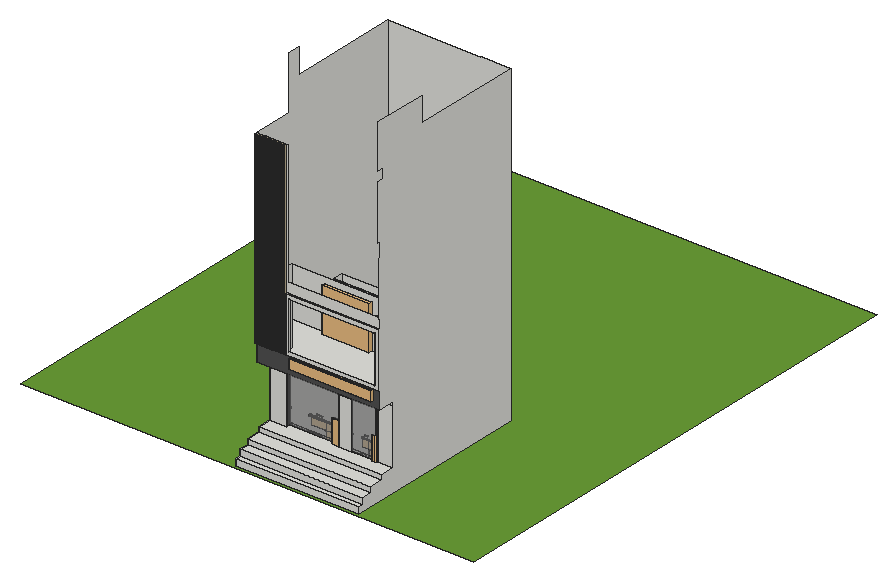
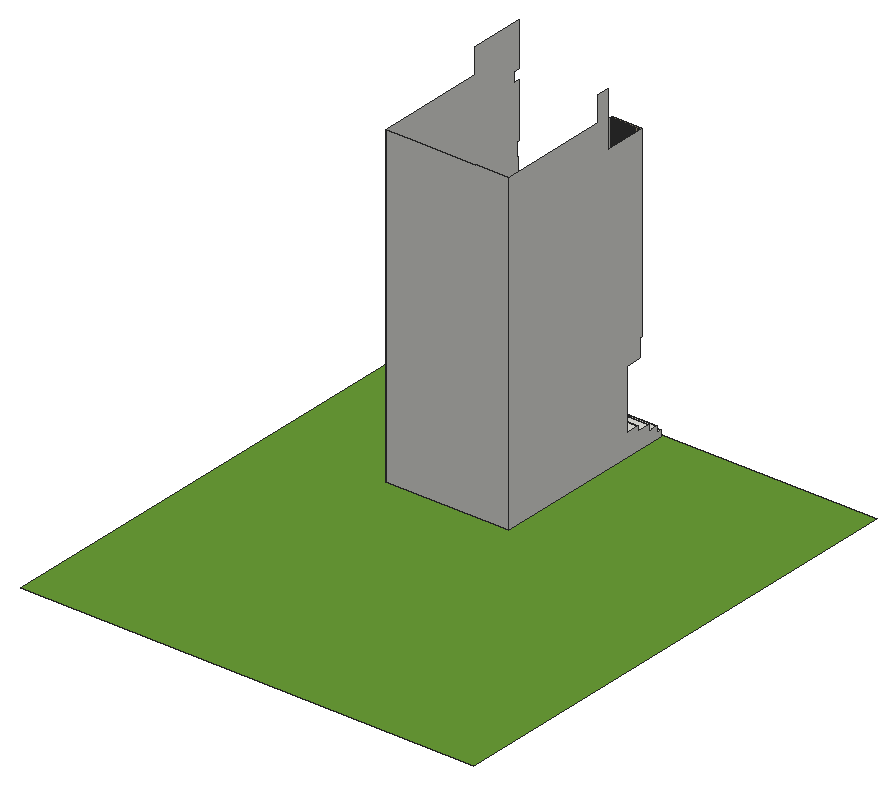
# SketchUp Ruby script. Lengths in inches.
U = 1.inch
M = Sketchup.active_model
def pt(a) = Geom::Point3d.new(a.map { |v| v * U })
def face(e, loops, mat)
  f = e.add_face(loops[0].map { |a| pt(a) })
  loops[1..].each { |l| e.add_face(l.map { |a| pt(a) }).erase! }
  f.material = f.back_material = mat if mat
  f
end
# faces: each face lists its corners as indices into pts; further lists are holes
def faces(e, pts, list, mat = nil) = list.each { |f| face(e, (f[0].is_a?(Array) ? f : [f]).map { |l| l.map { |i| pts[i] } }, mat) }
# xy, xz, yz: faces in a plane at the given z, y or x. An outline is a flat list of corners, or four numbers for a rectangle; further outlines are holes
def ring(l) = l.size == 4 ? [[l[0], l[1]], [l[2], l[1]], [l[2], l[3]], [l[0], l[3]]] : l.each_slice(2).to_a
def flat(e, list, mat, &to3) = list.each { |f| face(e, (f[0].is_a?(Array) ? f : [f]).map { |l| ring(l).map { |u, v| to3.(u, v) } }, mat) }
def xy(e, z, list, mat = nil) = flat(e, list, mat) { |x, y| [x, y, z] }
def xz(e, y, list, mat = nil) = flat(e, list, mat) { |x, z| [x, y, z] }
def yz(e, x, list, mat = nil) = flat(e, list, mat) { |y, z| [x, y, z] }
def lines(e, pts, list) = list.each { |a, b| e.add_line(pt(pts[a]), pt(pts[b])) }
# prism: a flat outline (further loops are holes) pulled along v
def prism(e, loops, v, mat = nil)
  f = face(e, loops, mat); d = Geom::Vector3d.new(v.map { |x| x * U })
  f.pushpull(f.normal.samedirection?(d) ? d.length : -d.length)
end
def box(e, o, s, mat = nil) = prism(e, [[o, [o[0] + s[0], o[1], o[2]], [o[0] + s[0], o[1] + s[1], o[2]], [o[0], o[1] + s[1], o[2]]]], [0, 0, s[2]], mat)
def at(x, y, z, deg = 0) = Geom::Transformation.translation(pt([x, y, z])) * Geom::Transformation.rotation(ORIGIN, Z_AXIS, deg.degrees)
def axes(o, x, y, z) = Geom::Transformation.new([*x, 0, *y, 0, *z, 0, *pt(o).to_a, 1])
def part(name) = M.definitions.add(name)
# library, detail: a bought-in or finely detailed component or shape, given as its bounding box
def library(name, o, s) = part(name).tap { |d| box(d.entities, o, s) }
def detail(e, o, s) = box(e.add_group.entities, o, s)
def put(e, d, t, mat = nil) = e.add_instance(d, t).tap { |i| i.material = mat if mat }
def group(e, t, mat = nil) = e.add_group.tap { |g| g.transformation = t; g.material = mat if mat }.entities
root = M.entities
M.materials.add("SW 0012 Empire Gold").color = [192, 162, 108]
M.materials.add("SW 0028 Caen Stone").color = [234, 212, 175]
M.materials.add("SW 0030 Colonial Yellow").color = [235, 202, 133]
M.materials.add("SW 0044 Hubbard Squash").color = [228, 196, 137]
M.materials.add("SW 0067 Belvedere Cream").color = [236, 208, 158]
M.materials.add("SW 0078 Sunbeam Yellow").color = [236, 216, 155]
M.materials.add("SW 2834 Birdseye Maple").color = [221, 199, 142]
M.materials.add("SW 2853 New Colonial Yellow").color = [211, 178, 125]
M.materials.add("SW 2857 Peace Yellow").color = [231, 210, 153]
M.materials.add("SW 2865 Classical Yellow").color = [244, 218, 144]
M.materials.add("SW 6113 Interactive Cream").color = [226, 206, 173]
M.materials.add("SW 6114 Bagel").color = [213, 185, 146]
M.materials.add("SW 6115 Totally Tan").color = [202, 170, 129]
M.materials.add("SW 6120 Believable Buff").color = [216, 202, 167]
M.materials.add("SW 6121 Whole Wheat").color = [203, 185, 145]
M.materials.add("SW 6122 Camelback").color = [194, 175, 133]
M.materials.add("SW 6127 Ivoire").color = [224, 209, 170]
M.materials.add("SW 6128 Blonde").color = [217, 193, 145]
M.materials.add("SW 6129 Restrained Gold").color = [206, 183, 131]
M.materials.add("SW 6134 Netsuke").color = [220, 210, 175]
M.materials.add("SW 6135 Ecru").color = [206, 193, 149]
M.materials.add("SW 6136 Harmonic Tan").color = [194, 179, 136]
M.materials.add("SW 6365 Cachet Cream").color = [240, 220, 183]
M.materials.add("SW 6366 Ambitious Amber").color = [238, 208, 148]
M.materials.add("SW 6372 Inviting Ivory").color = [239, 218, 175]
M.materials.add("SW 6373 Harvester").color = [232, 201, 137]
M.materials.add("SW 6379 Jersey Cream").color = [239, 224, 185]
M.materials.add("SW 6380 Humble Gold").color = [232, 206, 147]
M.materials.add("SW 6387 Compatible Cream").color = [229, 206, 156]
M.materials.add("SW 6388 Golden Fleece").color = [227, 182, 114]
M.materials.add("SW 6393 Convivial Yellow").color = [229, 218, 173]
M.materials.add("SW 6394 Sequin").color = [220, 200, 139]
M.materials.add("SW 6400 Lucent Yellow").color = [223, 213, 164]
M.materials.add("SW 6407 Ancestral Gold").color = [218, 210, 164]
M.materials.add("SW 6659 Captivating Cream").color = [243, 220, 176]
M.materials.add("SW 6660 Honey Blush").color = [243, 211, 152]
M.materials.add("SW 6666 Enjoyable Yellow").color = [244, 218, 167]
M.materials.add("SW 6667 Afterglow").color = [243, 209, 138]
M.materials.add("SW 6673 Banana Cream").color = [243, 226, 174]
M.materials.add("SW 6674 Jonquil").color = [244, 216, 142]
M.materials.add("SW 6680 Friendly Yellow").color = [241, 228, 176]
M.materials.add("SW 6681 Butter Up").color = [243, 225, 159]
M.materials.add("SW 6687 Lantern Light").color = [241, 228, 173]
M.materials.add("SW 6688 Solaria").color = [242, 221, 140]
M.materials.add("SW 6694 Glad Yellow").color = [240, 230, 169]
M.materials.add("SW 6701 Moonraker").color = [234, 231, 176]
M.materials.add("SW 6888 Pizazz Peach").color = [243, 202, 146]
M.materials.add("SW 6896 Solé").color = [243, 226, 157]
M.materials.add("SW 6900 Optimistic Yellow").color = [242, 228, 163]
M.materials.add("SW 6908 Fun Yellow").color = [242, 235, 145]
M.materials.add("SW 6912 Glisten Yellow").color = [240, 235, 169]
M.materials.add("SW 7537 Irish Cream").color = [227, 211, 186]
M.materials.add("SW 7676 Paper Lantern").color = [240, 224, 198]
M.materials.add("SW 7677 Gold Vessel").color = [233, 187, 138]
M.materials.add("SW 7678 Cottage Cream").color = [236, 219, 189]
M.materials.add("SW 7679 Golden Gate").color = [217, 176, 132]
M.materials.add("SW 7680 Lanyard").color = [191, 153, 116]
M.materials.add("SW 7681 Tea Light").color = [246, 227, 194]
M.materials.add("SW 7682 Bee_s Wax").color = [233, 192, 136]
M.materials.add("SW 7683 Buff").color = [242, 225, 197]
M.materials.add("SW 7684 Concord Buff").color = [239, 216, 182]
M.materials.add("SW 7685 White Raisin").color = [228, 192, 140]
M.materials.add("SW 7686 Hinoki").color = [246, 220, 183]
M.materials.add("SW 7687 August Moon").color = [231, 199, 161]
M.materials.add("SW 7688 Sundew").color = [223, 206, 176]
M.materials.add("SW 7689 Row House Tan").color = [211, 187, 159]
M.materials.add("SW 7690 Townhall Tan").color = [194, 171, 140]
M.materials.add("SW 7691 Biltmore Buff").color = [225, 202, 161]
M.materials.add("SW 7692 Cupola Yellow").color = [219, 188, 144]
M.materials.add("SW 7693 Stonebriar").color = [203, 172, 128]
M.materials.add("SW 7694 Dromedary Camel").color = [203, 175, 136]
M.materials.add("SW 7695 Mesa Tan").color = [190, 160, 124]
M.materials.add("SW 7696 Toasted Pine Nut").color = [218, 199, 167]
M.materials.add("SW 7697 Safari").color = [203, 179, 141]
M.materials.add("SW 7698 Straw Harvest").color = [217, 199, 161]
M.materials.add("SW 7717 Ligonier Tan").color = [211, 178, 143]
M.materials.add("Translucent_Glass_Gray1").color = [128, 128, 128]
M.materials["Translucent_Glass_Gray1"].alpha = 0.37
M.materials.add("[0010_Snow]").color = [255, 250, 250]
M.materials.add("[0135_DarkGray]").color = [81, 81, 81]
M.materials.add("[Color I05]").color = [0, 0, 255]
M.materials.add("[Grass Dark Green]").color = [106, 157, 55]
M.materials.add("[Quartz Light Brown]").color = [199, 184, 152]
M.materials.add("[Wax 01]").color = [250, 213, 163]
c1 = library("AED Menu Board with Easel",[149.1875,-32.32,34.05],[43.29,34.63,95.15])
c2 = part("Metal Door Roller Shutter")
xy(c2.entities,0,[[0,-0.5,0,4.5625,58.5,4.5625,58.5,-0.5,56.37,-0.5,56.37,1.125,1.83,1.125,1.83,-0.5]])
xy(c2.entities,0.79,[[22.59,1.375,35.41,4.1875]])
xy(c2.entities,1.04,[[2.77,1.125,54.9,1.375]])
xy(c2.entities,4.79,[[22.59,1.375,35.41,4.1875]])
xy(c2.entities,6.42,[[2.77,1.125,54.9,1.375]])
xy(c2.entities,116.14,[[1.83,0,56.37,1.125]])
xy(c2.entities,116.8,[[22.36,1.375,35.44,4.1875]])
xy(c2.entities,117.11,[[2.66,0,55.1,1.375]])
xy(c2.entities,119.36,[[2.66,0,55.1,1.375]])
xy(c2.entities,119.55,[[22.36,1.375,35.44,4.1875]])
xy(c2.entities,120.25,[[0,-0.5,1.83,-0.5,1.83,0,56.37,0,56.37,-0.5,58.5,-0.5,58.5,4.5625,0,4.5625]])
xz(c2.entities,-0.5,[[0,0,1.83,120.25],[56.37,0,58.5,120.25]])
xz(c2.entities,0,[[[1.83,116.14,56.37,120.25],[2.66,117.11,55.1,119.36]]])
xz(c2.entities,1.125,[[[1.83,0,56.37,116.14],[2.77,1.04,54.9,6.42]]])
xz(c2.entities,1.375,[[22.59,0.79,35.41,1.04],[2.77,1.04,22.59,1.04,22.59,4.79,35.41,4.79,35.41,1.04,54.9,1.04,54.9,6.42,2.77,6.42],[22.36,116.8,35.44,117.11],[2.66,117.11,22.36,119.36],[35.44,117.11,55.1,119.36],
  [22.36,119.36,35.44,119.55]])
xz(c2.entities,4.1875,[[22.59,0.79,35.41,4.79],[22.36,116.8,35.44,119.55]])
xz(c2.entities,4.5625,[[0,0,58.5,120.25]])
yz(c2.entities,0,[[-0.5,0,4.5625,120.25]])
yz(c2.entities,1.83,[[-0.5,0,1.125,0,1.125,116.14,0,116.14,0,120.25,-0.5,120.25]])
yz(c2.entities,2.66,[[0,117.11,1.375,119.36]])
yz(c2.entities,2.77,[[1.125,1.04,1.375,6.42]])
yz(c2.entities,22.36,[[1.375,116.8,4.1875,119.55]])
yz(c2.entities,22.59,[[1.375,0.79,4.1875,4.79]])
yz(c2.entities,35.41,[[1.375,0.79,4.1875,4.79]])
yz(c2.entities,35.44,[[1.375,116.8,4.1875,119.55]])
yz(c2.entities,54.9,[[1.125,1.04,1.375,6.42]])
yz(c2.entities,55.1,[[0,117.11,1.375,119.36]])
yz(c2.entities,56.37,[[-0.5,0,-0.5,120.25,0,120.25,0,116.14,1.125,116.14,1.125,0]])
yz(c2.entities,58.5,[[-0.5,0,4.5625,120.25]])
c3 = part("Metal Door Roller Shutter\#1")
put(c3.entities,c2,at(0,0,0),"Translucent_Glass_Gray1")
c4 = part("ROLLER+SHUTER+DOOR+VIEW")
yz(c4.entities,-109.06,[[2.88,0,9.21,28]],"[Color I05]")
yz(c4.entities,-108.56,[[43.65,14.75,44.44,15.25]])
yz(c4.entities,-108.56,[[51.96,34,67.8,35]],"[0010_Snow]")
yz(c4.entities,-108.56,[[9.21,2,43.65,14.75],[9.21,15.25,43.65,28],[44.44,15.25,78.88,28]],"[Wax 01]")
p = [[-109.06,85.21,28],[-109.04,85.21,28.26],[-109.04,2.88,28.26],[-109.06,2.88,28],[-109.06,9.21,28],[-109.06,129.55,28],
  [-109.03,129.55,28.26],[-109.03,135.88,28.26],[-109.06,135.88,28],[-108.99,85.21,28.52],[-108.99,2.88,28.52],[-108.96,129.55,28.5],
  [-108.96,135.88,28.5],[-108.91,85.21,28.77],[-108.91,2.88,28.77],[-108.87,129.55,28.74],[-108.87,135.88,28.74],[-108.75,129.55,28.97],
  [-108.75,135.88,28.97],[-108.79,85.21,29],[-108.79,2.88,29],[-108.65,85.21,29.22],[-108.65,2.88,29.22],[-108.6,129.55,29.18],
  [-108.6,135.88,29.18],[-108.47,85.21,29.42],[-108.47,2.88,29.42],[-108.43,129.55,29.375],[-108.43,135.88,29.375],[-108.28,85.21,29.59],
  [-108.28,2.88,29.59],[-108.24,129.55,29.55],[-108.24,135.88,29.55],[-108.03,129.55,29.69],[-108.03,135.88,29.69],[-108.06,85.21,29.73],
  [-108.06,2.88,29.73],[-107.82,85.21,29.85],[-107.82,2.88,29.85],[-107.8,129.55,29.8125],[-107.8,135.88,29.8125],[-107.58,85.21,29.93],
  [-107.58,2.88,29.93],[-107.5625,129.55,29.9],[-107.5625,135.88,29.9],[-107.32,85.21,29.98],[-107.32,2.88,29.98],[-107.3125,129.55,29.97],
  [-107.3125,135.88,29.97],[-107.06,85.21,30],[-107.06,2.88,30],[-107.06,129.55,30],[-107.06,135.88,30],[124.94,-3.12,0],
  [124.94,2.88,0],[-108.56,44.44,2],[-108.56,44.44,14.75],[-108.56,78.88,14.75]]
faces(c4.entities,p,[[0,1,2,3,4],[5,6,7,8],[1,9,10,2],[6,11,12,7],[9,13,14,10],[11,15,16,12],[15,17,18,16],[13,19,20,14],
  [19,21,22,20],[17,23,24,18],[21,25,26,22],[23,27,28,24],[25,29,30,26],[27,31,32,28],[31,33,34,32],[29,35,36,30],
  [35,37,38,36],[33,39,40,34],[37,41,42,38],[39,43,44,40],[41,45,46,42],[43,47,48,44],[45,49,50,46],[47,51,52,48]],"[0010_Snow]")
lines(c4.entities,p,[[53,54],[55,56],[57,56]])
put(c4.entities,c1,axes([-81.06,86.06,-14.77],[-0.19863,-0.42596,0],[0.32174,-0.15003,0],[0,0,0.43268]))
put(c4.entities,c3,axes([-114.53,135.88,0],[0,-2.2735,0],[1,0,0],[0,0,0.80749]))
c5 = library("XYZ  COMPLEX",[0.05,0,0],[86.34,9.9,1])
c6 = library("Group6\#1",[-22.44,-5.97,0],[42.52,9.29,84.25])
c7 = library("Spot Light",[-5.1,-5.1,-11.05],[10.2,10.2,11.05])
c8 = library("Glass_door",[70.54,1.5625,0],[78.74,7.87,82.68])
xy(root,0,[[1157.08,13.92,1824.45,1046.1]])
xy(root,0,[[[0,0,2460.75,2727],[1157.08,13.92,1824.45,1046.1]]],"[Grass Dark Green]")
xy(root,34.1,[[1157.08,13.92,1824.45,44.35]])
xy(root,68.21,[[1157.08,44.35,1824.45,97.98]])
xy(root,97.33,[[1157.08,97.98,1824.45,170.17]])
xy(root,121.875,[[1157.08,170.17,1824.45,170.17,1824.45,245.97,1740.62,245.97,1740.62,250.41,1598.85,250.41,1598.85,245.97,1532.65,245.97,1532.65,271.29,1246.76,271.29,1246.76,245.97,1157.08,245.97]])
xy(root,423.52,[[1246.76,245.97,1532.65,271.29],[1598.85,245.97,1740.62,250.41]])
xy(root,444.0625,[[1157.08,155.91,1246.76,245.97],[1246.76,155.91,1532.65,245.97],[1532.65,155.91,1598.85,245.97],[1598.85,155.91,1740.62,245.97],[1740.62,155.91,1824.45,245.97]])
xy(root,541.61,[[1157.08,144.72,1162.44,155.91],[1323.88,147.16,1324.61,155.91],[1324.61,147.16,1329.57,155.91],[1329.57,147.16,1337.99,155.91],[1337.99,147.16,1342.94,155.91],
  [1342.94,147.16,1351.36,155.91],[1351.36,147.16,1356.32,155.91],[1356.32,147.16,1364.74,155.91],[1364.74,147.16,1369.69,155.91],[1369.69,147.16,1378.11,155.91],
  [1378.11,147.16,1824.45,155.91]])
xy(root,541.61,[[1169.07,144.72,1177.49,155.91]],"[Quartz Light Brown]")
xy(root,558.56,[[1339.44,147.16,1805.83,147.16,1805.83,376.08,1604.22,376.08,1604.22,492.39,1349.53,492.39,1349.53,376.08,1169.07,376.08,1169.07,183.72,1324.51,183.72,1324.51,155.91,1339.44,155.91],[1323.88,147.16,1339.44,155.91]])
xz(root,13.92,[[1157.08,0,1824.45,34.1]])
xz(root,44.35,[[1157.08,34.1,1824.45,68.21]])
xz(root,97.98,[[1157.08,68.21,1824.45,97.33]])
xz(root,144.72,[[1157.08,541.61,1162.44,1555.875],[1169.07,541.61,1177.49,1555.875],[1182.44,541.61,1190.86,1555.875],[1195.82,541.61,1204.24,1555.875],[1209.19,541.61,1217.61,1555.875],
  [1222.57,541.61,1230.99,1555.875],[1235.94,541.61,1244.36,1555.875],[1249.32,541.61,1257.74,1555.875],[1262.69,541.61,1271.11,1555.875],[1276.07,541.61,1284.49,1555.875],
  [1289.44,541.61,1297.86,1555.875],[1302.82,541.61,1311.24,1555.875]])
xz(root,147.16,[[[1323.88,541.61,1824.45,836.67],[1339.44,558.56,1805.83,818.54]]])
xz(root,155.91,[[1316.19,541.61,1323.88,541.61,1323.88,836.67,1824.45,836.67,1824.45,889.6875,1324.51,889.6875,1324.51,1184.06,1324.16,1184.06,1324.16,1555.875,1316.19,1555.875],[1323.88,558.56,1324.51,827.6],[1324.51,558.56,1324.61,827.6],[1324.61,558.56,1329.57,827.6],[1329.57,558.56,1337.99,827.6],
  [1337.99,558.56,1337.99,827.6,1342.94,827.6,1342.94,818.54,1339.44,818.54,1339.44,558.56]])
xz(root,155.91,[[1157.08,444.0625,1824.45,541.61]],"[0135_DarkGray]")
xz(root,155.91,[[1162.44,541.61,1169.07,1555.875],[1177.49,541.61,1182.44,1555.875],[1182.44,541.61,1190.86,1555.875],[1190.86,541.61,1195.82,1555.875],[1195.82,541.61,1204.24,1555.875],
  [1204.24,541.61,1209.19,1555.875],[1209.19,541.61,1217.61,1555.875],[1217.61,541.61,1222.57,1555.875],[1222.57,541.61,1230.99,1555.875],[1230.99,541.61,1235.94,1555.875],
  [1235.94,541.61,1244.36,1555.875],[1244.36,541.61,1249.32,1555.875],[1249.32,541.61,1257.74,1555.875],[1257.74,541.61,1262.69,1555.875],[1262.69,541.61,1271.11,1555.875],
  [1271.11,541.61,1276.07,1555.875],[1276.07,541.61,1284.49,1555.875],[1284.49,541.61,1289.44,1555.875],[1289.44,541.61,1297.86,1555.875],[1297.86,541.61,1302.82,1555.875],
  [1302.82,541.61,1311.24,1555.875],[1311.24,541.61,1316.19,1555.875]],"[Quartz Light Brown]")
xz(root,170.17,[[1157.08,97.33,1824.45,121.875]])
xz(root,183.72,[[1169.07,558.56,1324.51,827.6]])
xz(root,245.97,[[1157.08,121.875,1246.76,423.52],[1532.65,121.875,1598.85,423.52],[1740.62,121.875,1824.45,423.52],[1157.08,423.52,1824.45,444.0625]])
xz(root,250.41,[[1598.85,121.875,1740.62,423.52]])
xz(root,271.29,[[1246.76,121.875,1532.65,423.52]])
xz(root,376.08,[[1169.07,558.56,1349.53,558.56,1349.53,793.31,1604.22,793.31,1604.22,558.56,1805.83,558.56,1805.83,827.6,1169.07,827.6]])
xz(root,434.23,[[[1358.03,557.61,1613.8,793.78],[1594.2,676.17,1612.85,694.82],[1358.98,676.17,1377.63,694.82],[1378.58,676.17,1397.23,694.82],[1398.18,676.17,1416.83,694.82],[1417.78,676.17,1436.43,694.82],[1437.38,676.17,1456.04,694.82],[1456.99,676.17,1475.64,694.82],[1476.59,676.17,1495.24,694.82],[1496.19,676.17,1514.84,694.82],[1515.79,676.17,1534.44,694.82],[1535.39,676.17,1554.05,694.82],[1555,676.17,1573.65,694.82],[1574.6,676.17,1593.25,694.82],[1594.2,656.57,1612.85,675.22],[1358.98,656.57,1377.63,675.22],[1378.58,656.57,1397.23,675.22],[1398.18,656.57,1416.83,675.22],[1417.78,656.57,1436.43,675.22],[1437.38,656.57,1456.04,675.22],[1456.99,656.57,1475.64,675.22],[1476.59,656.57,1495.24,675.22],[1496.19,656.57,1514.84,675.22],[1515.79,656.57,1534.44,675.22],[1535.39,656.57,1554.05,675.22],[1555,656.57,1573.65,675.22],[1574.6,656.57,1593.25,675.22],[1594.2,636.96,1612.85,655.62],[1594.2,695.77,1612.85,714.42],[1594.2,715.37,1612.85,734.02],[1594.2,734.97,1612.85,753.625],[1594.2,754.58,1612.85,773.23],[1594.2,558.56,1612.85,577.21],[1594.2,597.76,1612.85,616.41],[1358.98,754.58,1377.63,773.23],[1358.98,734.97,1377.63,753.625],[1358.98,715.37,1377.63,734.02],[1358.98,695.77,1377.63,714.42],[1358.98,636.96,1377.63,655.62],[1378.58,754.58,1397.23,773.23],[1378.58,734.97,1397.23,753.625],[1378.58,715.37,1397.23,734.02],[1378.58,695.77,1397.23,714.42],[1378.58,636.96,1397.23,655.62],[1398.18,636.96,1416.83,655.62],[1398.18,695.77,1416.83,714.42],[1398.18,715.37,1416.83,734.02],[1398.18,734.97,1416.83,753.625],[1398.18,754.58,1416.83,773.23],[1417.78,636.96,1436.43,655.62],[1417.78,695.77,1436.43,714.42],[1417.78,715.37,1436.43,734.02],[1417.78,734.97,1436.43,753.625],[1417.78,754.58,1436.43,773.23],[1594.2,578.16,1612.85,596.81],[1358.98,558.56,1377.63,577.21],[1378.58,558.56,1397.23,577.21],[1398.18,558.56,1416.83,577.21],[1417.78,558.56,1436.43,577.21],[1437.38,695.77,1456.04,714.42],[1437.38,636.96,1456.04,655.62],[1437.38,734.97,1456.04,753.625],[1437.38,754.58,1456.04,773.23],[1437.38,715.37,1456.04,734.02],[1456.99,754.58,1475.64,773.23],[1456.99,734.97,1475.64,753.625],[1456.99,715.37,1475.64,734.02],[1456.99,695.77,1475.64,714.42],[1456.99,636.96,1475.64,655.62],[1476.59,754.58,1495.24,773.23],[1476.59,734.97,1495.24,753.625],[1476.59,636.96,1495.24,655.62],[1476.59,695.77,1495.24,714.42],[1476.59,715.37,1495.24,734.02],[1496.19,636.96,1514.84,655.62],[1496.19,695.77,1514.84,714.42],[1496.19,715.37,1514.84,734.02],[1496.19,734.97,1514.84,753.625],[1496.19,754.58,1514.84,773.23],[1515.79,636.96,1534.44,655.62],[1515.79,695.77,1534.44,714.42],[1515.79,715.37,1534.44,734.02],[1515.79,734.97,1534.44,753.625],[1515.79,754.58,1534.44,773.23],[1535.39,636.96,1554.05,655.62],[1535.39,695.77,1554.05,714.42],[1535.39,715.37,1554.05,734.02],[1535.39,734.97,1554.05,753.625],[1535.39,754.58,1554.05,773.23],[1555,636.96,1573.65,655.62],[1555,695.77,1573.65,714.42],[1555,715.37,1573.65,734.02],[1555,734.97,1573.65,753.625],[1555,754.58,1573.65,773.23],[1574.6,636.96,1593.25,655.62],[1574.6,695.77,1593.25,714.42],[1574.6,715.37,1593.25,734.02],[1574.6,734.97,1593.25,753.625],[1574.6,754.58,1593.25,773.23],[1358.98,597.76,1377.63,616.41],[1378.58,597.76,1397.23,616.41],[1398.18,597.76,1416.83,616.41],[1417.78,597.76,1436.43,616.41],[1437.38,558.56,1456.04,577.21],[1456.99,558.56,1475.64,577.21],[1476.59,558.56,1495.24,577.21],[1496.19,558.56,1514.84,577.21],[1515.79,558.56,1534.44,577.21],[1535.39,558.56,1554.05,577.21],[1555,558.56,1573.65,577.21],[1574.6,558.56,1593.25,577.21],[1358.98,578.16,1377.63,596.81],[1378.58,578.16,1397.23,596.81],[1398.18,578.16,1416.83,596.81],[1417.78,578.16,1436.43,596.81],[1437.38,597.76,1456.04,616.41],[1456.99,597.76,1475.64,616.41],[1476.59,597.76,1495.24,616.41],[1496.19,597.76,1514.84,616.41],[1515.79,597.76,1534.44,616.41],[1535.39,597.76,1554.05,616.41],[1555,597.76,1573.65,616.41],[1574.6,597.76,1593.25,616.41],[1437.38,578.16,1456.04,596.81],[1456.99,578.16,1475.64,596.81],[1476.59,578.16,1495.24,596.81],[1496.19,578.16,1514.84,596.81],[1515.79,578.16,1534.44,596.81],[1535.39,578.16,1554.05,596.81],[1555,578.16,1573.65,596.81],[1574.6,578.16,1593.25,596.81],[1594.2,774.18,1612.85,792.83],[1594.2,617.36,1612.85,636.01],[1358.98,774.18,1377.63,792.83],[1358.98,617.36,1377.63,636.01],[1378.58,617.36,1397.23,636.01],[1378.58,774.18,1397.23,792.83],[1398.18,774.18,1416.83,792.83],[1398.18,617.36,1416.83,636.01],[1417.78,774.18,1436.43,792.83],[1417.78,617.36,1436.43,636.01],[1437.38,617.36,1456.04,636.01],[1437.38,774.18,1456.04,792.83],[1456.99,617.36,1475.64,636.01],[1456.99,774.18,1475.64,792.83],[1476.59,774.18,1495.24,792.83],[1476.59,617.36,1495.24,636.01],[1496.19,774.18,1514.84,792.83],[1496.19,617.36,1514.84,636.01],[1515.79,774.18,1534.44,792.83],[1515.79,617.36,1534.44,636.01],[1535.39,774.18,1554.05,792.83],[1535.39,617.36,1554.05,636.01],[1555,774.18,1573.65,792.83],[1555,617.36,1573.65,636.01],[1574.6,774.18,1593.25,792.83],[1574.6,617.36,1593.25,636.01]],[1574.6,558.56,1593.25,577.21],[1594.2,558.56,1612.85,577.21]])
xz(root,434.23,[[1476.59,656.57,1495.24,675.22]],"SW 0012 Empire Gold")
xz(root,434.23,[[1378.58,578.16,1397.23,596.81]],"SW 0028 Caen Stone")
xz(root,434.23,[[1358.98,597.76,1377.63,616.41]],"SW 0030 Colonial Yellow")
xz(root,434.23,[[1496.19,617.36,1514.84,636.01]],"SW 0044 Hubbard Squash")
xz(root,434.23,[[1456.99,617.36,1475.64,636.01]],"SW 0067 Belvedere Cream")
xz(root,434.23,[[1437.38,636.96,1456.04,655.62]],"SW 0078 Sunbeam Yellow")
xz(root,434.23,[[1574.6,656.57,1593.25,675.22]],"SW 2834 Birdseye Maple")
xz(root,434.23,[[1358.98,617.36,1377.63,636.01]],"SW 2853 New Colonial Yellow")
xz(root,434.23,[[1555,617.36,1573.65,636.01]],"SW 2857 Peace Yellow")
xz(root,434.23,[[1456.99,597.76,1475.64,616.41]],"SW 2865 Classical Yellow")
xz(root,434.23,[[1417.78,578.16,1436.43,596.81]],"SW 6113 Interactive Cream")
xz(root,434.23,[[1378.58,656.57,1397.23,675.22]],"SW 6114 Bagel")
xz(root,434.23,[[1358.98,656.57,1377.63,675.22]],"SW 6115 Totally Tan")
xz(root,434.23,[[1456.99,558.56,1475.64,577.21]],"SW 6120 Believable Buff")
xz(root,434.23,[[1456.99,636.96,1475.64,655.62]],"SW 6121 Whole Wheat")
xz(root,434.23,[[1476.59,636.96,1495.24,655.62]],"SW 6122 Camelback")
xz(root,434.23,[[1417.78,558.56,1436.43,577.21]],"SW 6127 Ivoire")
xz(root,434.23,[[1358.98,636.96,1377.63,655.62]],"SW 6128 Blonde")
xz(root,434.23,[[1378.58,636.96,1397.23,655.62]],"SW 6129 Restrained Gold")
xz(root,434.23,[[1476.59,558.56,1495.24,577.21]],"SW 6134 Netsuke")
xz(root,434.23,[[1515.79,636.96,1534.44,655.62]],"SW 6135 Ecru")
xz(root,434.23,[[1535.39,636.96,1554.05,655.62]],"SW 6136 Harmonic Tan")
xz(root,434.23,[[1398.18,578.16,1416.83,596.81]],"SW 6365 Cachet Cream")
xz(root,434.23,[[1417.78,617.36,1436.43,636.01]],"SW 6366 Ambitious Amber")
xz(root,434.23,[[1515.79,578.16,1534.44,596.81]],"SW 6372 Inviting Ivory")
xz(root,434.23,[[1476.59,617.36,1495.24,636.01]],"SW 6373 Harvester")
xz(root,434.23,[[1574.6,578.16,1593.25,596.81]],"SW 6379 Jersey Cream")
xz(root,434.23,[[1515.79,617.36,1534.44,636.01]],"SW 6380 Humble Gold")
xz(root,434.23,[[1358.98,558.56,1377.63,577.21]],"SW 6387 Compatible Cream")
xz(root,434.23,[[1594.2,656.57,1612.85,675.22]],"SW 6388 Golden Fleece")
xz(root,434.23,[[1496.19,558.56,1514.84,577.21]],"SW 6393 Convivial Yellow")
xz(root,434.23,[[1417.78,636.96,1436.43,655.62]],"SW 6394 Sequin")
xz(root,434.23,[[1535.39,558.56,1554.05,577.21]],"SW 6400 Lucent Yellow")
xz(root,434.23,[[1555,558.56,1573.65,577.21]],"SW 6407 Ancestral Gold")
xz(root,434.23,[[1378.58,617.36,1397.23,636.01]],"SW 6659 Captivating Cream")
xz(root,434.23,[[1437.38,617.36,1456.04,636.01]],"SW 6660 Honey Blush")
xz(root,434.23,[[1398.18,617.36,1416.83,636.01]],"SW 6666 Enjoyable Yellow")
xz(root,434.23,[[1574.6,617.36,1593.25,636.01]],"SW 6667 Afterglow")
xz(root,434.23,[[1594.2,617.36,1612.85,636.01]],"SW 6673 Banana Cream")
xz(root,434.23,[[1378.58,597.76,1397.23,616.41]],"SW 6674 Jonquil")
xz(root,434.23,[[1398.18,597.76,1416.83,616.41]],"SW 6680 Friendly Yellow")
xz(root,434.23,[[1437.38,597.76,1456.04,616.41]],"SW 6681 Butter Up")
xz(root,434.23,[[1476.59,597.76,1495.24,616.41]],"SW 6687 Lantern Light")
xz(root,434.23,[[1535.39,597.76,1554.05,616.41]],"SW 6688 Solaria")
xz(root,434.23,[[1555,597.76,1573.65,616.41]],"SW 6694 Glad Yellow")
xz(root,434.23,[[1358.98,578.16,1377.63,596.81]],"SW 6701 Moonraker")
xz(root,434.23,[[1574.6,636.96,1593.25,655.62]],"SW 6888 Pizazz Peach")
xz(root,434.23,[[1496.19,597.76,1514.84,616.41]],"SW 6896 Solé")
xz(root,434.23,[[1515.79,597.76,1534.44,616.41]],"SW 6900 Optimistic Yellow")
xz(root,434.23,[[1574.6,597.76,1593.25,616.41]],"SW 6908 Fun Yellow")
xz(root,434.23,[[1594.2,597.76,1612.85,616.41]],"SW 6912 Glisten Yellow")
xz(root,434.23,[[1437.38,578.16,1456.04,596.81]],"SW 7537 Irish Cream")
xz(root,434.23,[[1535.39,578.16,1554.05,596.81]],"SW 7676 Paper Lantern")
xz(root,434.23,[[1594.2,636.96,1612.85,655.62]],"SW 7677 Gold Vessel")
xz(root,434.23,[[1398.18,558.56,1416.83,577.21]],"SW 7678 Cottage Cream")
xz(root,434.23,[[1456.99,656.57,1475.64,675.22]],"SW 7679 Golden Gate")
xz(root,434.23,[[1437.38,656.57,1456.04,675.22]],"SW 7680 Lanyard")
xz(root,434.23,[[1496.19,578.16,1514.84,596.81]],"SW 7681 Tea Light")
xz(root,434.23,[[1535.39,617.36,1554.05,636.01]],"SW 7682 Bee_s Wax")
xz(root,434.23,[[1476.59,578.16,1495.24,596.81]],"SW 7683 Buff")
xz(root,434.23,[[1378.58,558.56,1397.23,577.21]],"SW 7684 Concord Buff")
xz(root,434.23,[[1417.78,597.76,1436.43,616.41]],"SW 7685 White Raisin")
xz(root,434.23,[[1594.2,578.16,1612.85,596.81]],"SW 7686 Hinoki")
xz(root,434.23,[[1555,578.16,1573.65,596.81]],"SW 7687 August Moon")
xz(root,434.23,[[1456.99,578.16,1475.64,596.81]],"SW 7688 Sundew")
xz(root,434.23,[[1398.18,656.57,1416.83,675.22]],"SW 7689 Row House Tan")
xz(root,434.23,[[1417.78,656.57,1436.43,675.22]],"SW 7690 Townhall Tan")
xz(root,434.23,[[1398.18,636.96,1416.83,655.62]],"SW 7691 Biltmore Buff")
xz(root,434.23,[[1555,656.57,1573.65,675.22]],"SW 7692 Cupola Yellow")
xz(root,434.23,[[1535.39,656.57,1554.05,675.22]],"SW 7693 Stonebriar")
xz(root,434.23,[[1515.79,656.57,1534.44,675.22]],"SW 7694 Dromedary Camel")
xz(root,434.23,[[1496.19,656.57,1514.84,675.22]],"SW 7695 Mesa Tan")
xz(root,434.23,[[1437.38,558.56,1456.04,577.21]],"SW 7696 Toasted Pine Nut")
xz(root,434.23,[[1496.19,636.96,1514.84,655.62]],"SW 7697 Safari")
xz(root,434.23,[[1515.79,558.56,1534.44,577.21]],"SW 7698 Straw Harvest")
xz(root,434.23,[[1555,636.96,1573.65,655.62]],"SW 7717 Ligonier Tan")
xz(root,492.39,[[1349.53,558.56,1604.22,793.31]])
xz(root,1046.1,[[1157.08,0,1157.08,1712.64,1330.44,1712.64,1330.44,1710.73,1668.23,1710.73,1668.23,1712.64,1824.45,1712.64,1824.45,0]])
yz(root,1157.08,[[13.92,0,13.92,34.1,44.35,34.1,44.35,68.21,97.98,68.21,97.98,97.33,170.17,97.33,170.17,121.875,245.97,121.875,245.97,444.0625,155.91,444.0625,155.91,541.61,144.72,541.61,144.72,1555.875,376.08,1555.875,376.08,1847.8125,440.47,1847.8125,440.47,1712.64,1046.1,1712.64,1046.1,0]])
yz(root,1162.44,[[144.72,541.61,155.91,1555.875]])
yz(root,1169.07,[[183.72,558.56,376.08,827.6]])
yz(root,1169.07,[[144.72,541.61,155.91,1555.875]],"[Quartz Light Brown]")
yz(root,1177.49,[[144.72,541.61,155.91,1555.875]],"[Quartz Light Brown]")
yz(root,1182.44,[[144.72,541.61,155.91,1555.875]],"[Quartz Light Brown]")
yz(root,1190.86,[[144.72,541.61,155.91,1555.875]],"[Quartz Light Brown]")
yz(root,1195.82,[[144.72,541.61,155.91,1555.875]],"[Quartz Light Brown]")
yz(root,1204.24,[[144.72,541.61,155.91,1555.875]],"[Quartz Light Brown]")
yz(root,1209.19,[[144.72,541.61,155.91,1555.875]],"[Quartz Light Brown]")
yz(root,1217.61,[[144.72,541.61,155.91,1555.875]],"[Quartz Light Brown]")
yz(root,1222.57,[[144.72,541.61,155.91,1555.875]],"[Quartz Light Brown]")
yz(root,1230.99,[[144.72,541.61,155.91,1555.875]],"[Quartz Light Brown]")
yz(root,1235.94,[[144.72,541.61,155.91,1555.875]],"[Quartz Light Brown]")
yz(root,1244.36,[[144.72,541.61,155.91,1555.875]],"[Quartz Light Brown]")
yz(root,1246.76,[[245.97,121.875,271.29,423.52]])
yz(root,1249.32,[[144.72,541.61,155.91,1555.875]],"[Quartz Light Brown]")
yz(root,1257.74,[[144.72,541.61,155.91,1555.875]],"[Quartz Light Brown]")
yz(root,1262.69,[[144.72,541.61,155.91,1555.875]],"[Quartz Light Brown]")
yz(root,1271.11,[[144.72,541.61,155.91,1555.875]],"[Quartz Light Brown]")
yz(root,1276.07,[[144.72,541.61,155.91,1555.875]],"[Quartz Light Brown]")
yz(root,1284.49,[[144.72,541.61,155.91,1555.875]],"[Quartz Light Brown]")
yz(root,1289.44,[[144.72,541.61,155.91,1555.875]],"[Quartz Light Brown]")
yz(root,1297.86,[[144.72,541.61,155.91,1555.875]],"[Quartz Light Brown]")
yz(root,1302.82,[[144.72,541.61,155.91,1555.875]],"[Quartz Light Brown]")
yz(root,1311.24,[[144.72,541.61,155.91,1555.875]],"[Quartz Light Brown]")
yz(root,1316.19,[[144.72,541.61,155.91,1555.875]],"[Quartz Light Brown]")
yz(root,1323.88,[[147.16,541.61,155.91,558.56],[147.16,558.56,155.91,836.67]])
yz(root,1324.51,[[155.91,558.56,183.72,827.6]])
yz(root,1339.44,[[147.16,558.56,155.91,818.54]])
yz(root,1349.53,[[376.08,558.56,492.39,793.31]])
yz(root,1532.65,[[245.97,121.875,271.29,423.52]])
yz(root,1598.85,[[245.97,121.875,250.41,423.52]])
yz(root,1604.22,[[376.08,558.56,492.39,756.91]])
yz(root,1740.62,[[245.97,121.875,250.41,423.52]])
yz(root,1805.83,[[147.16,558.56,147.16,818.54,155.91,818.54,155.91,827.6,376.08,827.6,376.08,558.56]])
yz(root,1824.45,[[13.92,0,1046.1,0,1046.1,1712.64,440.47,1712.64,440.47,1847.8125,143.16,1847.8125,143.16,1610.73,176.1,1610.73,176.1,1555.875,143.16,1555.875,143.16,1262.78,154.6,1262.78,154.6,1184.06,147.66,1184.06,147.66,889.6875,155.91,889.6875,155.91,836.67,147.16,836.67,147.16,541.61,155.91,541.61,155.91,444.0625,245.97,444.0625,245.97,121.875,170.17,121.875,170.17,97.33,97.98,97.33,97.98,68.21,44.35,68.21,44.35,34.1,13.92,34.1]])
p = [[1775.37,376.08,731.61],[1775.37,376.08,558.56],[1324.61,144.72,541.61],[1316.19,144.72,541.61],[1324.61,155.91,558.56],[1324.61,155.91,541.61],
  [1324.61,147.16,541.61],[1329.57,155.91,541.61],[1329.57,155.91,558.56],[1337.99,144.72,541.61],[1329.57,144.72,541.61],[1337.99,155.91,558.56],
  [1337.99,155.91,541.61],[1337.99,147.16,541.61],[1329.57,147.16,541.61],[1351.36,144.72,541.61],[1342.94,144.72,541.61],[1351.36,147.16,541.61],
  [1342.94,147.16,541.61],[1364.74,144.72,541.61],[1356.32,144.72,541.61],[1364.74,147.16,541.61],[1356.32,147.16,541.61],[1378.11,144.72,541.61],
  [1369.69,144.72,541.61],[1378.11,147.16,541.61],[1369.69,147.16,541.61]]
lines(root,p,[[0,1],[2,3],[4,5],[6,2],[7,8],[9,10],[11,12],[13,9],[14,10],[15,16],[17,15],[18,16],
  [19,20],[21,19],[22,20],[23,24],[25,23],[26,24]])
put(root,c4,axes([1548.63,331.99,121.875],[0,0.66323,0],[-2.22156,0,0],[0,0,3.06]))
put(root,c4,axes([1739.31,294.51,122.01],[0,0.43521,0],[-1.01816,0,0],[0,0,3.06]))
put(root,c5,axes([1338.6,155.91,476.84],[5.16672,0,0],[0,0,5.16672],[0,-10.90178,0]))
put(root,c6,axes([1705.13,380.02,514.18],[3.3125,0,0],[0,1.0865,0],[0,0,2.65]))
put(root,c7,at(1352.14,155.57,537.82))
put(root,c7,at(1477.64,155.57,537.82))
put(root,c7,at(1612.39,155.57,537.82))
put(root,c7,at(1702.29,155.57,537.82))
put(root,c8,axes([1119.28,353.45,558.56],[3.264,0,0],[0,2.4,0],[0,0,2.86214]))
